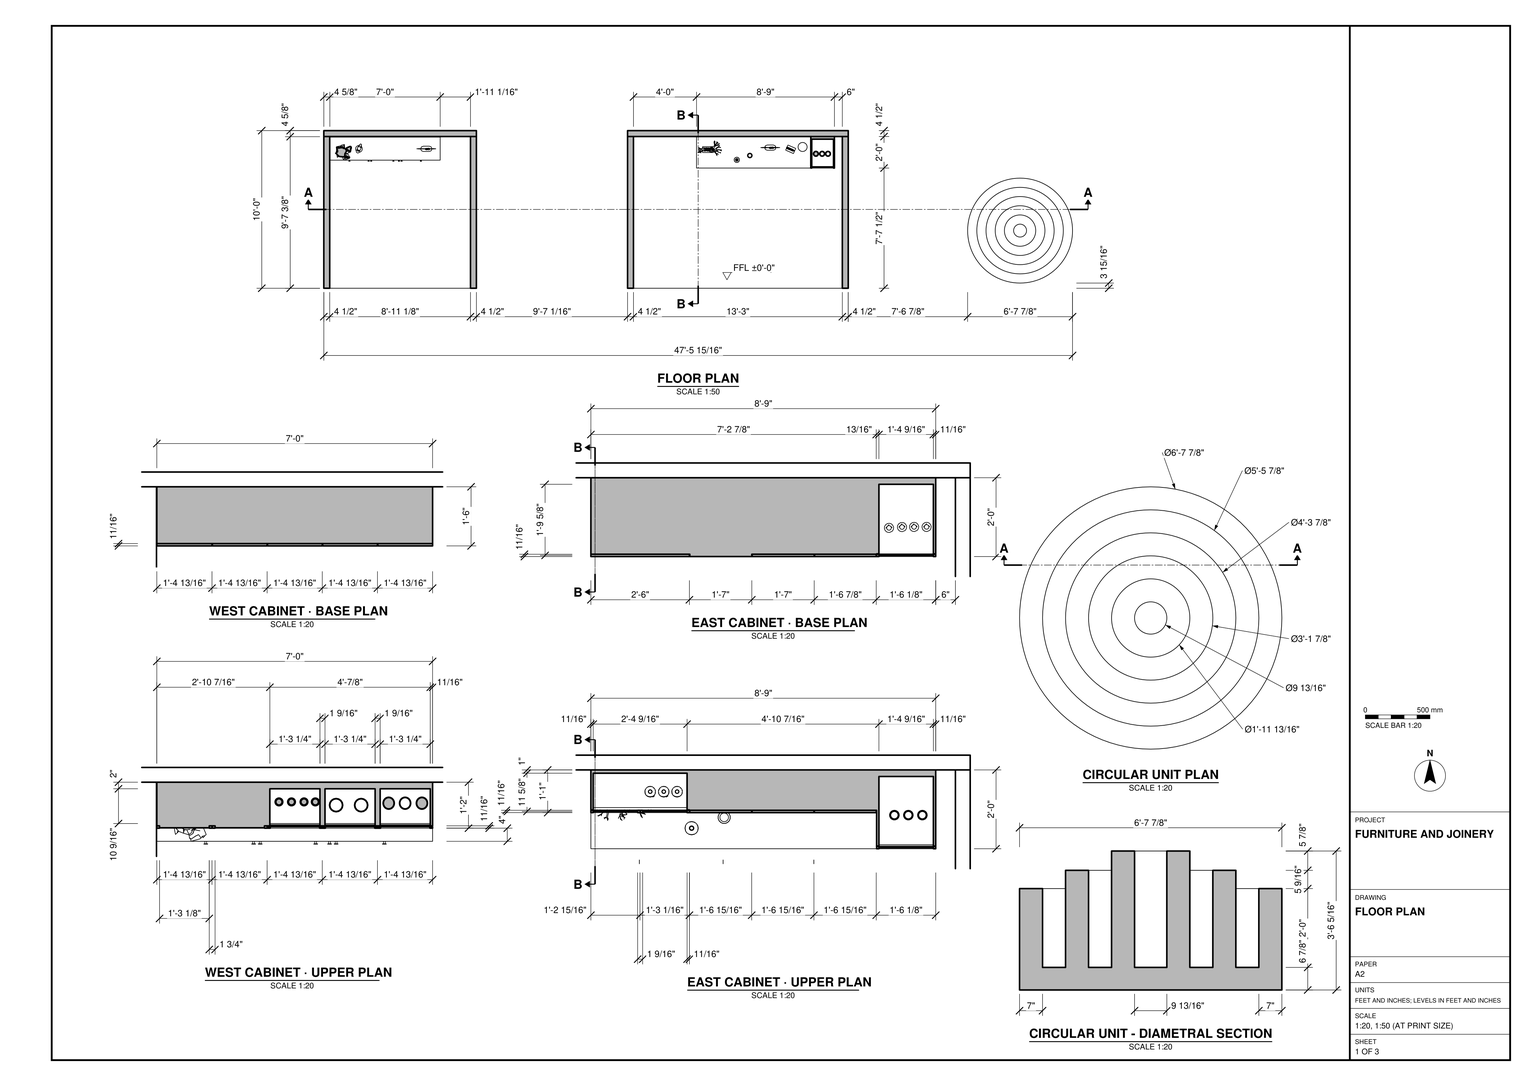
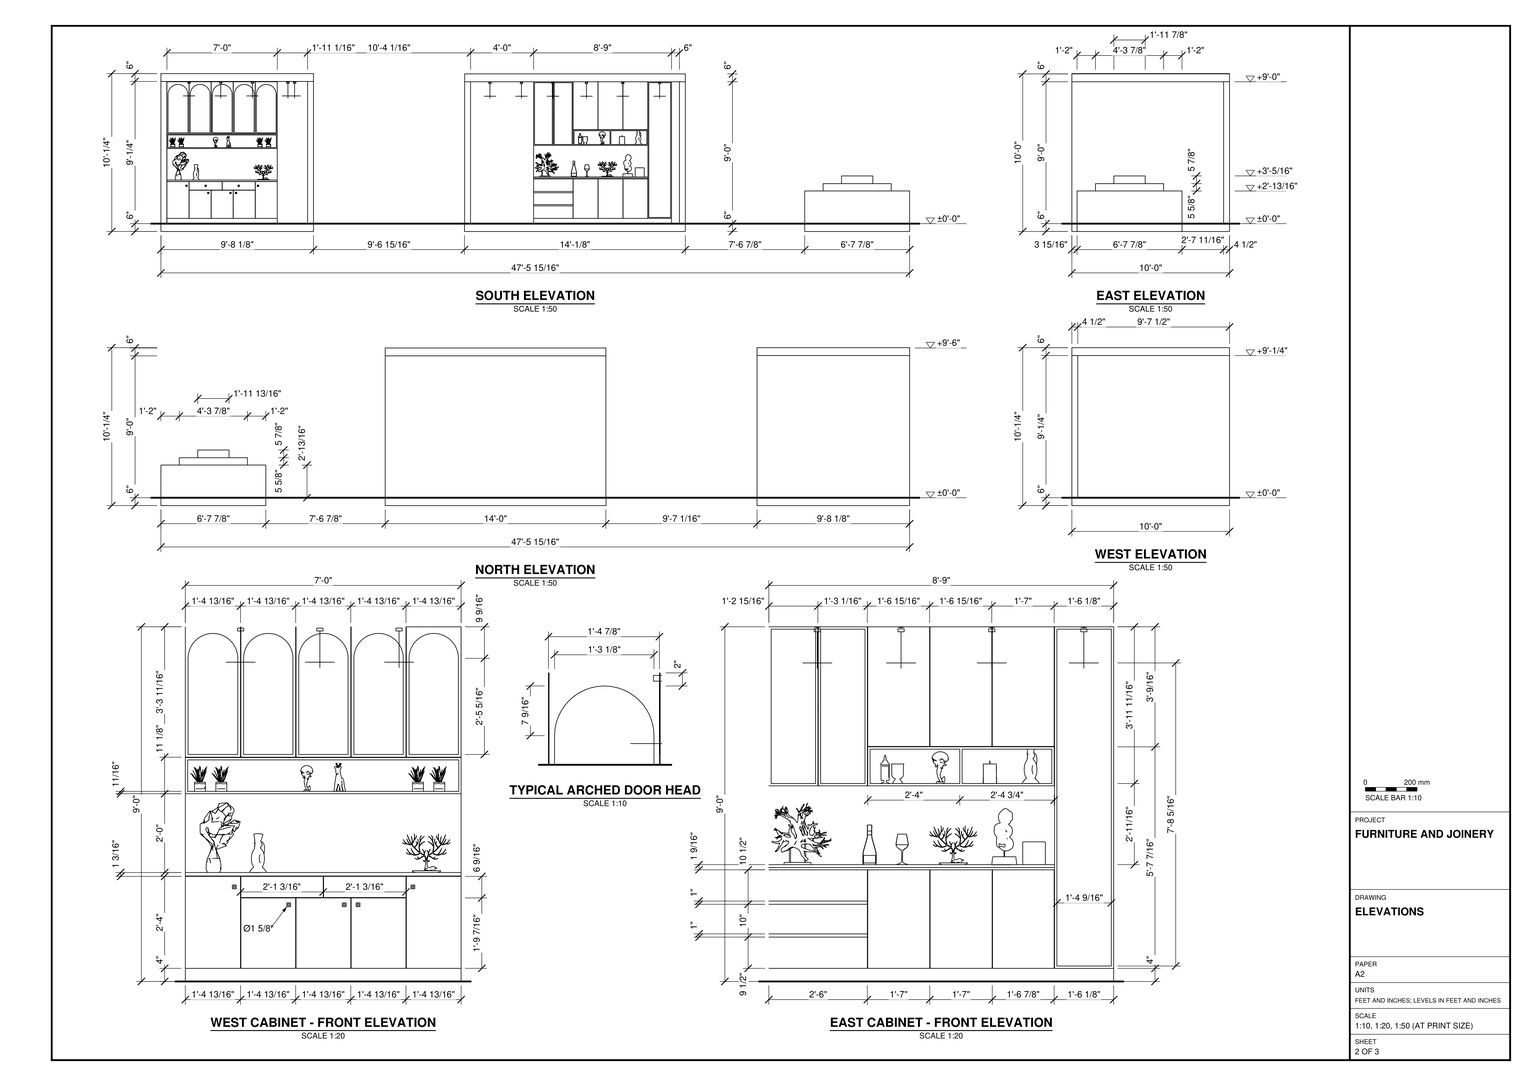
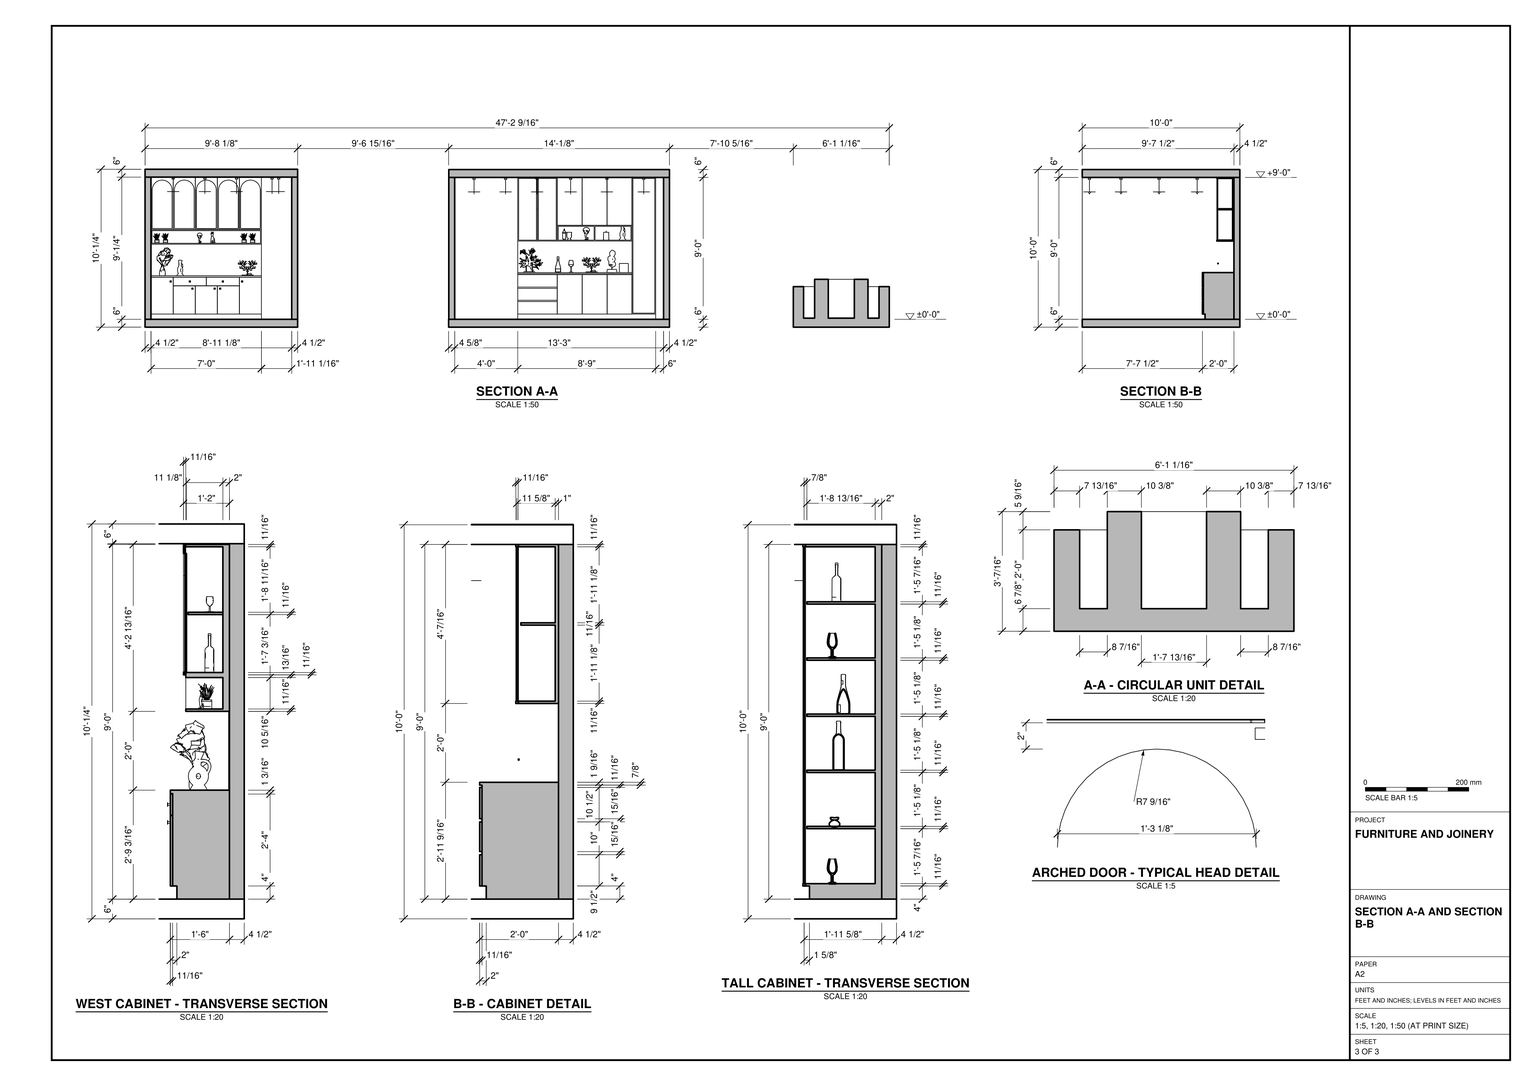
Work in feet and inches in SketchUp. Use task_files/diagram_01.pdf to model the west and east cabinet displays and the freestanding circular unit. Set the finished floor level to ±0'-0". The complete arrangement is 47'-5 15/16" long, 10'-0" deep and 10'-1/4" high.

Build each cabinet bay with a back wall, side walls, floor slab and overhead slab, leaving the south face open. Follow the wall and slab thicknesses in plan and section. Fit the 7'-0" west cabinet against the back wall at the left end of its bay. Model the recessed plinth, base doors and drawers, countertop, open display shelf and five arched upper door details. In the wider bay, leave 4'-0" of clear wall to the left of the 8'-9" east cabinet. Include the drawer bank, base doors, rectangular upper cupboards, open display compartments and full-height shelved cabinet at the right end.

Place the circular unit beyond the east bay. Use the diametral section to form its concentric walls on a common base, with open channels between the walls and the highest rim nearest the centre. Decor and loose items, including plants, bottles, glasses and ornaments, may be any suitable library components placed on the indicated counters and shelves.

Keep shell elements and each joinery piece in separate groups or components, and use components for repeated parts. Save one SketchUp model as output_files/two_cabinet_displays_and_freestanding_circular_unit.skp.

# SketchUp Ruby script. Lengths in inches.
U = 1.inch
M = Sketchup.active_model
def pt(a) = Geom::Point3d.new(a.map { |v| v * U })
def face(e, loops, mat)
  f = e.add_face(loops[0].map { |a| pt(a) })
  loops[1..].each { |l| e.add_face(l.map { |a| pt(a) }).erase! }
  f.material = f.back_material = mat if mat
  f
end
# faces: each face lists its corners as indices into pts; further lists are holes
def faces(e, pts, list, mat = nil) = list.each { |f| face(e, (f[0].is_a?(Array) ? f : [f]).map { |l| l.map { |i| pts[i] } }, mat) }
# xy, xz, yz: faces in a plane at the given z, y or x. An outline is a flat list of corners, or four numbers for a rectangle; further outlines are holes
def ring(l) = l.size == 4 ? [[l[0], l[1]], [l[2], l[1]], [l[2], l[3]], [l[0], l[3]]] : l.each_slice(2).to_a
def flat(e, list, mat, &to3) = list.each { |f| face(e, (f[0].is_a?(Array) ? f : [f]).map { |l| ring(l).map { |u, v| to3.(u, v) } }, mat) }
def xy(e, z, list, mat = nil) = flat(e, list, mat) { |x, y| [x, y, z] }
def xz(e, y, list, mat = nil) = flat(e, list, mat) { |x, z| [x, y, z] }
def yz(e, x, list, mat = nil) = flat(e, list, mat) { |y, z| [x, y, z] }
def lines(e, pts, list) = list.each { |a, b| e.add_line(pt(pts[a]), pt(pts[b])) }
# prism: a flat outline (further loops are holes) pulled along v
def prism(e, loops, v, mat = nil)
  f = face(e, loops, mat); d = Geom::Vector3d.new(v.map { |x| x * U })
  f.pushpull(f.normal.samedirection?(d) ? d.length : -d.length)
end
def box(e, o, s, mat = nil) = prism(e, [[o, [o[0] + s[0], o[1], o[2]], [o[0] + s[0], o[1] + s[1], o[2]], [o[0], o[1] + s[1], o[2]]]], [0, 0, s[2]], mat)
def at(x, y, z, deg = 0) = Geom::Transformation.translation(pt([x, y, z])) * Geom::Transformation.rotation(ORIGIN, Z_AXIS, deg.degrees)
def axes(o, x, y, z) = Geom::Transformation.new([*x, 0, *y, 0, *z, 0, *pt(o).to_a, 1])
def part(name) = M.definitions.add(name)
# library, detail: a bought-in or finely detailed component or shape, given as its bounding box
def library(name, o, s) = part(name).tap { |d| box(d.entities, o, s) }
def detail(e, o, s) = box(e.add_group.entities, o, s)
def put(e, d, t, mat = nil) = e.add_instance(d, t).tap { |i| i.material = mat if mat }
def group(e, t, mat = nil) = e.add_group.tap { |g| g.transformation = t; g.material = mat if mat }.entities
root = M.entities
M.materials.add("Sublime-734-Blanc-White-4K").color = [233, 236, 235]
M.materials.add("Sublime-735-Vert-Relax-Relax-Green-4K").color = [135, 152, 141]
M.materials.add("Uniboard-L17-Ambrette-4K").color = [104, 52, 49]
M.materials.add("Uniboard-L19-Putty-4K").color = [187, 181, 160]
M.materials.add("[Color M09]").color = [0, 0, 0]
M.materials.add("[Translucent Glass Gray]").color = [128, 128, 128]
M.materials["[Translucent Glass Gray]"].alpha = 0.5
c1 = library("Decoration 111 063",[-2.51,-1.28,-0.03],[5.02,2.53,10.66])
c2 = library("Interior Props 221 030",[-2.57,-3.63,-0.04],[5.13,7.27,11.89])
c3 = library("Decorative Jar 83-09",[-5.58,-3.02,0],[11.21,6.04,13.74])
c4 = library("Candle 111 040",[-2.11,-2.13,-0.02],[4.23,4.26,6.92])
c5 = library("Stand 298 006",[-6.74,-6.74,-0.04],[13.48,13.48,13.7])
c6 = library("Interior Props 221 024",[-3.28,-2.14,-0.05],[6.56,4.27,17.12])
c7 = library("Tree Decoration 83-10",[-18.61,-13.07,0],[43.1,29.04,44.77])
c8 = library("Decorative Deer 97-30",[-7.23,-2.03,0],[14.46,4,11.8125])
c9 = library("Wine Bottle 03 87-10",[-1.625,-1.66,0],[3.25,3.3,10.61])
c10 = library("Glass 002",[-1.85,-1.85,0.02],[3.7,3.7,9.27])
c11 = library("Bottle 05 87-12",[-2.04,-2.04,0],[4.08,4.08,12.09])
c12 = library("2-PRODUITS CUISINE CLC2",[-1.33,-1.33,0],[2.66,2.66,10.8])
c13 = library("16-PRODUITS CUISINE CLC2",[-2.49,-2.49,0],[4.98,4.98,4.3])
c14 = library("Vases 04 65-25",[-1.8125,-1.8125,0],[3.625,3.625,14.95])
c15 = part("Group39\#1")
p = [[0,0,0],[0,0,-2.67],[-1.27,0,-2.67],[8.29,-0.35,0],[-8.29,-0.35,0],[8.29,0.35,0],
  [8.29,0,0],[-8.29,0.35,0],[1.27,0,-2.67],[-8.29,0,0],[0,0,-4.32]]
lines(c15.entities,p,[[0,1],[1,2],[3,4],[5,6],[7,5],[1,8],[9,0],[0,6],[8,10],[4,9],[6,3],[2,10],
  [9,7]])
c16 = part("Rectangle Light")
put(c16.entities,c15,at(0,0,0))
c17 = part("Group41\#1")
p = [[0,0,0],[0,0,-13.54],[-6.68,0,-13.54],[43.5,-0.34,0],[-43.5,-0.34,0],[43.5,0.34,0],
  [43.5,0,0],[-43.5,0.34,0],[6.68,0,-13.54],[-43.5,0,0],[0,0,-21.92]]
lines(c17.entities,p,[[0,1],[1,2],[3,4],[5,6],[7,5],[1,8],[9,0],[0,6],[8,10],[4,9],[6,3],[2,10],
  [9,7]])
c18 = part("Rectangle Light\#1")
put(c18.entities,c17,at(0,0,0))
c19 = part("Group43\#1")
p = [[0,0,0],[0,0,-4.52],[-2.2,0,-4.52],[14.29,-0.35,0],[-14.29,-0.35,0],[14.29,0.35,0],
  [14.29,0,0],[-14.29,0.35,0],[2.2,0,-4.52],[-14.29,0,0],[0,0,-7.32]]
lines(c19.entities,p,[[0,1],[1,2],[3,4],[5,6],[7,5],[1,8],[9,0],[0,6],[8,10],[4,9],[6,3],[2,10],
  [9,7]])
c20 = part("Rectangle Light\#2")
put(c20.entities,c19,at(0,0,0))
c21 = part("Group45\#1")
p = [[0,0,0],[0,0,-4.33],[-2.1,0,-4.33],[13.66,-0.35,0],[-13.66,-0.35,0],[13.66,0.35,0],
  [13.66,0,0],[-13.66,0.35,0],[2.1,0,-4.33],[-13.66,0,0],[0,0,-7.01]]
lines(c21.entities,p,[[0,1],[1,2],[3,4],[5,6],[7,5],[1,8],[9,0],[0,6],[8,10],[4,9],[6,3],[2,10],
  [9,7]])
c22 = part("Rectangle Light\#3")
put(c22.entities,c21,at(0,0,0))
c23 = library("Wine 193 001",[-1.36,-1.37,-0.03],[2.74,2.77,11.85])
c24 = library("Wine Bottle 01 87-10",[-1.37,-1.39,0],[2.74,2.78,10.53])
c25 = library("Glass 298 004 004",[-1.29,-1.29,-0.01],[2.58,2.58,4.79])
c26 = part("Group68\#1")
p = [[0,0,0],[0,0,-2.47],[-1.17,0,-2.47],[7.63,-0.35,0],[-7.63,-0.35,0],[7.63,0.35,0],
  [7.63,0,0],[-7.63,0.35,0],[1.17,0,-2.47],[-7.63,0,0],[0,0,-3.99]]
lines(c26.entities,p,[[0,1],[1,2],[3,4],[5,6],[7,5],[1,8],[9,0],[0,6],[8,10],[4,9],[6,3],[2,10],
  [9,7]])
c27 = part("Rectangle Light\#4")
put(c27.entities,c26,at(0,0,0))
c28 = library("Interior Plant 273 003 001",[-15.3,-29.38,0],[45.32,44.44,78.66])
c29 = library("Decorative Deer 209 004",[-1.58,-4.16,0],[3.36,7.25,10.63])
c30 = library("Potted Succulent 003",[-4.09,-3.62,0],[7.1,6.83,10.79])
c31 = part("Group73\#1")
p = [[0,0,0],[0,0,-12.86],[-6.34,0,-12.86],[41.28,-0.35,0],[-41.28,-0.35,0],[41.28,0.35,0],
  [41.28,0,0],[-41.28,0.35,0],[6.34,0,-12.86],[-41.28,0,0],[0,0,-20.82]]
lines(c31.entities,p,[[0,1],[1,2],[3,4],[5,6],[7,5],[1,8],[9,0],[0,6],[8,10],[4,9],[6,3],[2,10],
  [9,7]])
c32 = part("Rectangle Light\#5")
put(c32.entities,c31,at(0,0,0))
c33 = library("031",[-37.9375,-66.55,25.1875],[1.17,0.87,1.16])
c34 = library("Wine Glass 293 011",[-1.4,-1.42,-0.1],[2.82,2.8,7.63])
c35 = library("Group\#6",[0,0,0],[8.9,8.9,12.63])
c36 = part("Group\#8")
box(c36.entities,[3.84,0,0],[116.16,120,6])
c37 = library("Group\#11",[0,4,0],[83.97,14,50.82])
c38 = library("Group\#18",[0,0,0],[8.9,8.9,12.63])
xz(root,91.85,[[371.43,10.71,388.01,113.29]],"[Translucent Glass Gray]")
detail(root,[490.09,3.96,0],[79.88,79.87,42.3125])
put(root,c1,axes([335.9,107.74,66.28],[1,0,0],[0,1,0],[0,0,0.91]))
put(root,c2,at(363.56,107.74,66.28,-21.7))
put(root,c3,axes([321.28,107.85,66.28],[0.63,0,0],[0,0.63,0],[0,0,0.63]))
put(root,c4,at(351.03,106.9,66.28))
put(root,c5,axes([364.47,107.5625,41.55],[0.51,0,0],[0,0.51,0],[0,0,0.51]))
put(root,c6,at(355.37,105.8125,41.57,-23.6))
put(root,c7,axes([292.47,105.56,41.57],[0.42,0,0],[0,0.42,0],[0,0,0.42]))
put(root,c8,at(339.87,107.08,41.57))
put(root,c9,at(309.96,108.875,90.14))
put(root,c9,at(305.9,108.875,90.14))
put(root,c9,at(301.77,108.875,90.14))
put(root,c10,at(324.31,101.05,41.57))
put(root,c11,at(314.39,97.76,41.57))
put(root,c11,at(384.35,103.82,62.35))
put(root,c11,at(379.41,103.82,62.35))
put(root,c11,at(374.35,103.82,62.35))
put(root,c12,at(287.78,109.78,90.14))
put(root,c12,at(291.4,109.78,90.14))
put(root,c12,at(295.03,109.78,90.14))
put(root,c13,at(376.64,101.11,27.63))
put(root,c13,at(383.33,101.11,27.63))
put(root,c14,at(379.35,102.37,45.26))
put(root,c14,at(374.6,102.37,45.26))
put(root,c14,at(383.79,102.37,45.26))
put(root,c16,axes([379.72,112.4375,113.28],[1,0,0],[0,-1,0],[0,0,1]))
put(root,c16,axes([379.72,112.4375,95.84],[1,0,0],[0,-1,0],[0,0,1]))
put(root,c16,axes([379.72,112.4375,78.74],[1,0,0],[0,-1,0],[0,0,1]))
put(root,c16,axes([379.72,112.4375,61.65],[1,0,0],[0,-1,0],[0,0,1]))
put(root,c16,axes([379.72,112.4375,44.55],[1,0,0],[0,-1,0],[0,0,1]))
put(root,c16,axes([379.72,112.4375,27.45],[1,0,0],[0,-1,0],[0,0,1]))
put(root,c18,at(327.22,114.45,65.56,180))
put(root,c20,at(298.72,112.4375,113.28,180))
put(root,c20,at(298.72,112.4375,89.42,180))
put(root,c22,axes([328.2,113.4375,76.74],[1,0,0],[0,-1,0],[0,0,1]))
put(root,c22,axes([356.23,113.4375,76.74],[1,0,0],[0,-1,0],[0,0,1]))
put(root,c23,at(41.98,109.39,75.01))
put(root,c23,at(46.36,109.39,75.01))
put(root,c23,at(50.79,109.39,75.01))
put(root,c24,at(58.8,108.51,75.01))
put(root,c24,at(63.68,108.51,75.01))
put(root,c24,at(68.43,108.51,75.01))
put(root,c9,at(75.77,109.55,75.01))
put(root,c9,at(80.2,109.55,75.01))
put(root,c9,at(85.08,109.55,75.01))
put(root,c25,at(41.79,109.5,93.36))
put(root,c25,at(45.61,109.5,93.36))
put(root,c25,at(49.42,109.5,93.36))
put(root,c25,at(52.86,109.5,93.36))
put(root,c14,axes([75.21,109.11,93.36],[0.94,0,0],[0,1,0],[0,0,0.89]))
put(root,c14,axes([80.2,109.11,93.36],[0.94,0,0],[0,1,0],[0,0,0.89]))
put(root,c14,axes([85.32,109.11,93.36],[0.94,0,0],[0,1,0],[0,0,0.89]))
put(root,c11,at(59.19,108.51,93.36))
put(root,c11,at(66.82,108.51,93.36))
put(root,c27,at(46.65,106.69,113.28,180))
put(root,c27,at(63.44,105.88,113.28,180))
put(root,c27,at(80.24,105.38,113.28,180))
put(root,c27,at(80.24,105.94,92.64,180))
put(root,c27,at(46.65,107.69,92.64,180))
put(root,c27,at(63.44,105.94,92.64,180))
put(root,c28,axes([13.22,105.43,39.18],[0.27,0,0],[0,0.27,0],[0,0,0.27]))
put(root,c1,axes([41.57,107.05,63.88],[0.74,0,0],[0,0.74,0],[0,0,0.74]))
put(root,c2,at(26.85,106.41,39.18,-23.2))
put(root,c29,axes([51.47,108.15,63.89],[0.7824,-0.20964,0],[0.20964,0.7824,0],[0,0,0.81]))
put(root,c8,at(78.01,106.17,39.18))
put(root,c30,axes([9.08,108.55,63.89],[0.71,0,0],[0,0.71,0],[0,0,0.71]))
put(root,c30,axes([15.58,108.55,63.89],[0.71,0,0],[0,0.71,0],[0,0,0.71]))
put(root,c30,axes([75.46,108.55,63.89],[0.71,0,0],[0,0.71,0],[0,0,0.71]))
put(root,c30,axes([81.96,108.55,63.89],[0.71,0,0],[0,0.71,0],[0,0,0.71]))
put(root,c32,axes([46.59,112.4375,73.46],[1,0,0],[0,-1,0],[0,0,1]))
put(root,c32,axes([47.3,114.4375,63.17],[1,0,0],[0,-1,0],[0,0,1]))
put(root,c33,at(71.43,163.18,9.03))
put(root,c33,at(96.55,163.18,9.03))
put(root,c33,at(94.55,163.18,3.59))
put(root,c33,at(73.43,163.18,3.59))
put(root,c33,at(90.33,163.18,3.59))
put(root,c33,at(111.24,163.18,9.03))
put(root,c33,at(56.86,163.18,9.03))
g1 = group(root,at(279.22,0,0))
box(g1,[-48.12,0,0],[168.12,120,6])
g2 = group(root,at(279.22,115.5,6))
xy(g2,0,[[-47.99,0,120,4.5]])
xy(g2,108,[[-47.99,0,120,4.5]])
xz(g2,0,[[-47.99,0,4.5,108],[4.5,0,115.5,0,115.5,108,4.5,108,4.5,59.57,91.5,59.57,91.5,35.57,4.5,35.57],[115.5,0,120,108],[4.5,35.57,91.5,59.57]])
xz(g2,4.5,[[-47.99,0,120,108]])
yz(g2,-47.99,[[0,0,4.5,108]])
yz(g2,120,[[0,0,4.5,108]])
g3 = group(root,at(283.72,91.5,6),"Uniboard-L19-Putty-4K")
xy(g3,0,[[0,2,87,24],[87,2,105,24]])
xy(g3,4,[[0,0,30,0.71],[30.12,0,49,0.71],[49.12,0,68,0.71],[68.12,0,86.88,0.71],[87,0,105,0.71],
  [0,0.71,30,2],[30,0.71,49,2],[49,0.71,68,2],[68,0.71,87,2],[87,0.83,105,2]])
xy(g3,4.71,[[87.71,0.83,104.29,22]],"Uniboard-L17-Ambrette-4K")
xy(g3,4.71,[[87.71,0,104.29,0.71]],"[Color M09]")
xy(g3,13.51,[[0,0,30,0.71]],"[Color M09]")
xy(g3,14.49,[[0,0,30,0.71]],"[Color M09]")
xy(g3,21.45,[[87.71,1.22,104.29,22]],"Uniboard-L17-Ambrette-4K")
xy(g3,22.16,[[87.71,1.22,104.29,22]],"Uniboard-L17-Ambrette-4K")
xy(g3,23.51,[[0,0,30,0.71]],"[Color M09]")
xy(g3,24.49,[[0,0,30,0.71]],"[Color M09]")
xy(g3,34,[[0,0,30,0.71],[30.12,0,49,0.71],[49.12,0,68,0.71],[68.12,0,86.88,0.71]])
xy(g3,34.71,[[0,0,87,0.71]])
xy(g3,35.57,[[0,0,87,24]])
xy(g3,38.55,[[87.71,1.22,104.29,22]],"Uniboard-L17-Ambrette-4K")
xy(g3,39.26,[[87.71,1.22,104.29,22]],"Uniboard-L17-Ambrette-4K")
xy(g3,55.65,[[87.71,1.22,104.29,22]],"Uniboard-L17-Ambrette-4K")
xy(g3,56.35,[[87.71,1.22,104.29,22]],"Uniboard-L17-Ambrette-4K")
xy(g3,59.57,[[0,11,14.94,11.71],[15.06,11,30,11.71],[30.12,11.52,30.12,11.71,30,11.71,30,11.83,0,11.83,0,24,87,24,87,11.71,86.88,11.71,86.88,11.52]])
xy(g3,60.28,[[30.83,11.52,58.15,23],[58.85,11.52,86.17,23],[0.71,11.83,29.29,23]],"Uniboard-L17-Ambrette-4K")
xy(g3,60.28,[[0.71,11,14.23,11.35],[15.77,11,29.29,11.35],[0.71,11.35,14.23,11.71],[15.77,11.35,29.29,11.71]],"[Color M09]")
xy(g3,70.75,[[30.83,11.52,58.15,23],[58.85,11.52,86.17,23]],"Uniboard-L17-Ambrette-4K")
xy(g3,71.46,[[67.92,11.52,68.04,11.71]])
xy(g3,71.46,[[30.12,11.52,48.96,11.71],[48.96,11.52,49.08,11.71],[49.08,11.52,67.92,11.71],[68.04,11.52,86.88,11.71]],"Uniboard-L17-Ambrette-4K")
xy(g3,71.57,[[30.12,11,48.96,11.71],[49.08,11,67.92,11.71],[68.04,11,86.88,11.71]])
xy(g3,72.74,[[87.71,1.22,104.29,22]],"Uniboard-L17-Ambrette-4K")
xy(g3,73.45,[[87.71,1.22,104.29,22]],"Uniboard-L17-Ambrette-4K")
xy(g3,83.43,[[0.71,12.54,29.29,23]],"Uniboard-L17-Ambrette-4K")
xy(g3,84.14,[[0.71,12.54,29.29,23]],"Uniboard-L17-Ambrette-4K")
xy(g3,89.84,[[87.71,1.22,104.29,22]],"Uniboard-L17-Ambrette-4K")
xy(g3,90.55,[[87.71,1.22,104.29,22]],"Uniboard-L17-Ambrette-4K")
xy(g3,107.29,[[87.71,0.83,104.29,22],[0.71,11.83,29.29,23]],"Uniboard-L17-Ambrette-4K")
xy(g3,107.29,[[87.71,0,104.29,0.71],[0.71,11,14.23,11.35],[15.77,11,29.29,11.35],[0.71,11.35,14.23,11.71],[15.77,11.35,29.29,11.71]],"[Color M09]")
xy(g3,108,[[87,0.83,105,0.83,105,24,0,24,0,11.83,30,11.83,30,11.71,87,11.71],[30.12,11,48.96,11.71],[49.08,11,67.92,11.71],[68.04,11,86.88,11.71]])
xy(g3,108,[[87,0,105,0.71],[0,11,14.94,11.71],[15.06,11,30,11.71]],"[Color M09]")
xz(g3,0,[[0,4,30,13.51],[30.12,4,49,34],[49.12,4,68,34],[68.12,4,86.88,34],[0,14.49,30,23.51],
  [0,24.49,30,34],[0,34.71,87,35.57]])
xz(g3,0,[[[87,4,105,108],[87.71,4.71,104.29,107.29]]],"[Color M09]")
xz(g3,0.71,[[0,4,30,13.51],[30,4,30.12,34],[49,4,49.12,34],[49.12,4,68,34],[68,4,68.12,34],
  [68.12,4,86.88,34],[86.88,4,87,34],[87,4,104.29,4.71],[104.29,4,105,108],[87,4.71,87.71,107.29],
  [0,14.49,30,23.51],[0,24.49,30,34],[87,107.29,104.29,108]])
xz(g3,0.71,[[0,13.51,30,14.49],[0,23.51,30,24.49],[0,34,87,34.71]],"[Color M09]")
xz(g3,0.83,[[87,4,104.29,4.71],[104.29,4,105,108],[87,4.71,87.71,107.29],[87,107.29,104.29,108]],"Uniboard-L17-Ambrette-4K")
xz(g3,1.22,[[87.71,21.45,104.29,22.16],[87.71,38.55,104.29,39.26],[87.71,55.65,104.29,56.35],[87.71,72.74,104.29,73.45],[87.71,89.84,104.29,90.55]],"Uniboard-L17-Ambrette-4K")
xz(g3,2,[[0,0,105,4]])
xz(g3,11,[[30.12,71.57,48.96,108],[68.04,71.57,86.88,108]])
xz(g3,11,[[49.08,71.57,67.92,108]],"Uniboard-L19-Putty-4K")
xz(g3,11,[[[0,59.57,14.94,108],[0.71,60.28,14.23,107.29]],[[15.06,59.57,30,108],[15.77,60.28,29.29,107.29]]],"[Color M09]")
xz(g3,11.35,[[0.71,60.28,14.23,107.29],[15.77,60.28,29.29,107.29]],"[Translucent Glass Gray]")
xz(g3,11.52,[[[30.12,59.57,86.88,71.46],[30.83,60.28,58.15,70.75],[58.85,60.28,86.17,70.75]]],"Uniboard-L17-Ambrette-4K")
xz(g3,11.71,[[0,59.57,0.71,108],[0.71,59.57,14.94,60.28],[15.06,59.57,30,60.28],[30,59.57,30.12,108],[86.88,59.57,87,108],
  [14.23,60.28,14.23,107.29,0.71,107.29,0.71,108,14.94,108,14.94,60.28],[15.06,60.28,15.06,108,29.29,108,29.29,107.29,15.77,107.29,15.77,60.28],[29.29,60.28,30,108],[30.12,71.46,86.88,71.57],[30.12,71.57,48.96,108],
  [48.96,71.57,49.08,108],[49.08,71.57,67.92,108],[67.92,71.57,68.04,108],[68.04,71.57,86.88,108]])
xz(g3,11.83,[[0,59.57,30,59.57,30,60.28,0.71,60.28,0.71,107.29,29.29,107.29,29.29,60.28,30,60.28,30,108,0,108]],"Uniboard-L17-Ambrette-4K")
xz(g3,12.54,[[0.71,83.43,29.29,84.14]],"Uniboard-L17-Ambrette-4K")
xz(g3,22,[[87.71,4.71,104.29,21.45],[87.71,22.16,104.29,38.55],[87.71,39.26,104.29,55.65],[87.71,56.35,104.29,72.74],[87.71,73.45,104.29,89.84],
  [87.71,90.55,104.29,107.29]],"Uniboard-L17-Ambrette-4K")
xz(g3,23,[[0.71,60.28,29.29,83.43],[30.83,60.28,58.15,70.75],[58.85,60.28,86.17,70.75],[0.71,84.14,29.29,107.29]],"Uniboard-L17-Ambrette-4K")
xz(g3,24,[[0,0,87,34],[87,0,87,59.57,0,59.57,0,108,105,108,105,0],[0,34,87,35.57]])
yz(g3,0,[[2,0,2,4,0.71,4,0.71,34.71,24,34.71,24,0],[0,4,0.71,13.51],[0,14.49,0.71,23.51],[0,24.49,0.71,34],[0,34.71,24,35.57],
  [11.83,59.57,24,108]])
yz(g3,0,[[11,59.57,11.71,108]],"[Color M09]")
yz(g3,0.71,[[11.83,60.28,23,60.28,23,83.43,12.54,83.43,12.54,84.14,23,84.14,23,107.29,11.83,107.29]],"Uniboard-L17-Ambrette-4K")
yz(g3,0.71,[[11,60.28,11.35,107.29],[11.35,60.28,11.71,107.29]],"[Color M09]")
yz(g3,14.23,[[11,60.28,11.35,107.29],[11.35,60.28,11.71,107.29]],"[Color M09]")
yz(g3,14.94,[[11,59.57,11.71,108]],"[Color M09]")
yz(g3,15.06,[[11,59.57,11.71,108]],"[Color M09]")
yz(g3,15.77,[[11,60.28,11.35,107.29],[11.35,60.28,11.71,107.29]],"[Color M09]")
yz(g3,29.29,[[11.83,60.28,11.83,107.29,23,107.29,23,84.14,12.54,84.14,12.54,83.43,23,83.43,23,60.28]],"Uniboard-L17-Ambrette-4K")
yz(g3,29.29,[[11,60.28,11.35,107.29],[11.35,60.28,11.71,107.29]],"[Color M09]")
yz(g3,30,[[0,4,0.71,13.51],[0,14.49,0.71,23.51],[0,24.49,0.71,34],[11.71,59.57,11.83,108]])
yz(g3,30,[[11,59.57,11.71,108]],"[Color M09]")
yz(g3,30.12,[[0,4,0.71,34],[11.52,59.57,11.71,71.46],[11,71.57,11.71,108]])
yz(g3,30.83,[[11.52,60.28,23,70.75]],"Uniboard-L17-Ambrette-4K")
yz(g3,48.96,[[11,71.57,11.71,108]])
yz(g3,49,[[0,4,0.71,34]])
yz(g3,49.08,[[11,71.57,11.71,108]])
yz(g3,49.12,[[0,4,0.71,34]])
yz(g3,58.15,[[11.52,60.28,23,70.75]],"Uniboard-L17-Ambrette-4K")
yz(g3,58.85,[[11.52,60.28,23,70.75]],"Uniboard-L17-Ambrette-4K")
yz(g3,67.92,[[11,71.57,11.71,108]])
yz(g3,68,[[0,4,0.71,34]])
yz(g3,68.04,[[11,71.57,11.71,108]])
yz(g3,68.12,[[0,4,0.71,34]])
yz(g3,86.17,[[11.52,60.28,23,70.75]],"Uniboard-L17-Ambrette-4K")
yz(g3,86.88,[[0,4,0.71,34],[11,71.57,11.71,108]])
yz(g3,86.88,[[11.52,59.57,11.71,71.46]],"Uniboard-L17-Ambrette-4K")
yz(g3,87,[[0,4,0.71,34],[0.71,4,0.83,34],[0,34,0.71,34.71],[0.71,34,0.83,35.57],[0.83,34,24,35.57],
  [0,34.71,0.71,35.57],[0.71,35.57,0.83,108],[0.83,35.57,0.83,108,11.71,108,11.71,59.57,24,59.57,24,35.57]])
yz(g3,87,[[0,35.57,0.71,108]],"[Color M09]")
yz(g3,87.71,[[0.83,4.71,22,4.71,22,21.45,1.22,21.45,1.22,22.16,22,22.16,22,38.55,1.22,38.55,1.22,39.26,22,39.26,22,55.65,1.22,55.65,1.22,56.35,22,56.35,22,72.74,1.22,72.74,1.22,73.45,22,73.45,22,89.84,1.22,89.84,1.22,90.55,22,90.55,22,107.29,0.83,107.29]],"Uniboard-L17-Ambrette-4K")
yz(g3,87.71,[[0,4.71,0.71,107.29]],"[Color M09]")
yz(g3,104.29,[[0.83,4.71,0.83,107.29,22,107.29,22,90.55,1.22,90.55,1.22,89.84,22,89.84,22,73.45,1.22,73.45,1.22,72.74,22,72.74,22,56.35,1.22,56.35,1.22,55.65,22,55.65,22,39.26,1.22,39.26,1.22,38.55,22,38.55,22,22.16,1.22,22.16,1.22,21.45,22,21.45,22,4.71]],"Uniboard-L17-Ambrette-4K")
yz(g3,104.29,[[0,4.71,0.71,107.29]],"[Color M09]")
yz(g3,105,[[2,0,24,0,24,108,0.83,108,0.83,4,2,4]])
yz(g3,105,[[0,4,0.71,108]],"[Color M09]")
put(g3,c23,at(26.86,17.26,60.28))
put(g3,c34,at(3.14,17.62,60.28))
put(g3,c34,at(6.98,17.87,60.28))
put(g3,c34,at(10.34,17.91,60.28))
put(g3,c23,at(22.59,17.26,60.28))
put(g3,c23,at(18.34,17.26,60.28))
put(g3,c34,at(94.73,8.99,4.71))
put(g3,c34,at(98.41,9.02,4.71))
put(g3,c34,at(90.77,8.73,4.71))
put(g3,c34,at(102.22,9.02,4.71))
put(g3,c23,at(100.93,10.21,90.55))
put(g3,c23,at(92.41,10.21,90.55))
put(g3,c23,at(96.66,10.21,90.55))
put(g3,c34,at(98.41,9.02,73.45))
put(g3,c34,at(94.73,8.99,73.45))
put(g3,c34,at(90.77,8.73,73.45))
put(g3,c34,at(102.22,9.02,73.45))
g4 = group(root,at(231.22,0,6))
box(g4,[0,0,0],[4.5,115.5,108])
g5 = group(root,at(394.72,0,6))
box(g5,[0,0,0],[4.5,115.5,108])
g6 = group(root,at(279.22,0,114))
box(g6,[-47.99,0,0],[167.99,120,6])
put(root,c35,at(294.02,83.05,101.37))
put(root,c35,at(319.53,83.05,101.37))
put(root,c35,at(347.16,83.05,101.37))
put(root,c35,at(375.19,70.25,101.37))
put(root,c35,at(347.16,54.05,101.37))
put(root,c35,at(319.53,54.05,101.37))
put(root,c35,at(294.02,54.05,101.37))
put(root,c35,at(347.16,25.05,101.37))
put(root,c35,at(319.53,25.05,101.37))
put(root,c35,at(294.02,25.05,101.37))
put(root,c35,at(347.16,1.05,101.37))
put(root,c35,at(319.53,1.05,101.37))
put(root,c35,at(294.02,1.05,101.37))
put(root,c35,at(375.19,46.25,101.37))
put(root,c35,at(375.19,22.25,101.37))
put(root,c35,at(375.19,2.44,101.37))
put(root,c35,at(270.02,1.05,101.37))
put(root,c35,at(270.02,25.05,101.37))
put(root,c35,at(270.02,83.05,101.37))
put(root,c35,at(270.02,54.05,101.37))
put(root,c35,at(246.02,1.05,101.37))
put(root,c35,at(246.02,25.05,101.37))
put(root,c35,at(246.02,83.05,101.37))
put(root,c35,at(246.02,54.05,101.37))
put(root,c35,at(246.02,103.05,101.37))
put(root,c35,at(270.02,103.05,101.37))
put(root,c36,at(-3.84,0,0))
g7 = group(root,at(-3.84,115.5,6))
xy(g7,0,[[3.84,0,120,4.5]])
xy(g7,33.18,[[8.44,-0.12,92.42,0]])
xy(g7,57.18,[[8.44,-0.12,92.42,0]])
xy(g7,108.24,[[3.84,0,120,4.5]])
xz(g7,-0.12,[[8.44,33.18,92.42,57.18]])
xz(g7,0,[[[3.84,0,120,108.24],[8.44,33.18,92.42,57.18]],[8.44,33.18,92.42,57.18]])
xz(g7,4.5,[[3.84,0,120,108.24]])
yz(g7,3.84,[[0,0,4.5,108.24]])
yz(g7,8.44,[[-0.12,33.18,0,57.18]])
yz(g7,92.42,[[-0.12,33.18,0,57.18]])
yz(g7,120,[[0,0,4.5,108.24]])
g8 = group(root,at(4.6,97.5,6),"Sublime-734-Blanc-White-4K")
xy(g8,0,[[0,2,83.97,18]])
xy(g8,4,[[0,0,16.79,0.71],[16.91,0,33.59,0.71],[33.71,0,50.38,0.71],[50.5,0,67.18,0.71],[67.3,0,83.97,0.71],
  [0,0.71,83.97,2]])
xy(g8,25.44,[[16.91,0,33.59,0.71],[33.71,0,50.38,0.71],[50.5,0,67.18,0.71]])
xy(g8,25.56,[[16.91,0,41.99,0.71],[42.11,0,67.18,0.71]])
xy(g8,32,[[0,0,16.79,0.71],[16.91,0,33.59,0.71],[33.59,0,41.99,0.71],[42.11,0,50.38,0.71],[50.38,0,67.18,0.71],
  [67.3,0,83.97,0.71]])
xy(g8,32.12,[[0,0,83.97,0.71]],"Sublime-735-Vert-Relax-Relax-Green-4K")
xy(g8,33.18,[[0,0,83.97,18]],"Sublime-735-Vert-Relax-Relax-Green-4K")
xz(g8,0,[[0,4,16.79,32],[16.91,4,33.59,25.44],[33.71,4,50.38,25.44],[50.5,4,67.18,25.44],[67.3,4,83.97,32],
  [16.91,25.56,41.99,32],[42.11,25.56,67.18,32]])
xz(g8,0,[[0,32.12,83.97,33.18]],"Sublime-735-Vert-Relax-Relax-Green-4K")
xz(g8,0.71,[[0,4,16.79,32],[16.79,4,16.91,32],[16.91,4,33.59,25.44],[33.59,4,33.71,25.44],[33.71,4,50.38,25.44],
  [50.38,4,50.5,25.44],[50.5,4,67.18,25.44],[67.18,4,67.3,32],[67.3,4,83.97,32],[16.91,25.44,67.18,25.44,67.18,25.56,42.11,25.56,42.11,32,41.99,32,41.99,25.56,16.91,25.56],
  [16.91,25.56,41.99,32],[42.11,25.56,67.18,32],[0,32,83.97,32.12]])
xz(g8,2,[[0,0,83.97,4]],"Sublime-735-Vert-Relax-Relax-Green-4K")
xz(g8,18,[[0,0,83.97,32],[0,32,83.97,33.18]])
yz(g8,0,[[2,0,2,4,0.71,4,0.71,32.12,18,32.12,18,0],[0,4,0.71,32],[0,32.12,18,33.18]])
yz(g8,16.79,[[0,4,0.71,25.44],[0,25.44,0.71,32]])
yz(g8,16.91,[[0,4,0.71,25.44],[0,25.56,0.71,32]])
yz(g8,33.59,[[0,4,0.71,25.44]])
yz(g8,33.71,[[0,4,0.71,25.44]])
yz(g8,41.99,[[0,25.56,0.71,32]])
yz(g8,42.11,[[0,25.56,0.71,32]])
yz(g8,50.38,[[0,4,0.71,25.44]])
yz(g8,50.5,[[0,4,0.71,25.44]])
yz(g8,67.18,[[0,4,0.71,25.44],[0,25.56,0.71,32]])
yz(g8,67.3,[[0,4,0.71,32]])
yz(g8,83.97,[[2,0,18,0,18,32.12,0.71,32.12,0.71,4,2,4],[0,4,0.71,32]])
yz(g8,83.97,[[0,32.12,18,33.18]],"Sublime-735-Vert-Relax-Relax-Green-4K")
put(root,c37,at(4.6,97.5,63.18),"Sublime-735-Vert-Relax-Relax-Green-4K")
g9 = group(root,at(39.02,102.92,92.65),"Sublime-735-Vert-Relax-Relax-Green-4K")
box(g9,[0,0,0],[15.26,10.58,0.71])
box(g9,[33.59,0,0],[15.26,10.58,0.71])
xy(g9,0,[[16.79,0,32.05,10.58]],"Sublime-735-Vert-Relax-Relax-Green-4K")
xy(g9,0.71,[[16.79,0,32.05,10.58]],"Sublime-735-Vert-Relax-Relax-Green-4K")
xz(g9,0,[[16.79,0,32.05,0.71]],"Sublime-735-Vert-Relax-Relax-Green-4K")
xz(g9,10.58,[[16.79,0,32.05,0.71]])
yz(g9,16.79,[[0,0,10.58,0.71]])
yz(g9,32.05,[[0,0,10.58,0.71]])
g10 = group(root,at(0,0,6))
box(g10,[0,0,0],[4.5,115.5,108.24])
g11 = group(root,at(38.31,101.5,74.3),"Sublime-735-Vert-Relax-Relax-Green-4K")
xy(g11,0,[[0,0,16.68,0.46]])
xy(g11,0.83,[[0.83,0,15.85,0.92]])
xy(g11,39.7,[[0,0,16.68,0.46]])
xz(g11,0,[[[0,0,16.68,39.7],[0.83,0.83,15.85,0.83,15.85,30.1875,15.79,31.17,15.59,32.13,15.28,33.0625,14.84,33.95,14.3,34.76,13.65,35.5,12.91,36.15,12.09,36.69,11.21,37.13,10.28,37.44,9.32,37.64,8.34,37.7,7.36,37.64,6.39,37.44,5.46,37.13,4.58,36.69,3.77,36.15,3.03,35.5,2.38,34.76,1.83,33.95,1.4,33.0625,1.08,32.13,0.89,31.17,0.83,30.1875]]])
xz(g11,0.46,[[0,0,16.68,39.7]],"[Translucent Glass Gray]")
xz(g11,0.92,[[0.83,0.83,0.83,30.1875,0.89,31.17,1.08,32.13,1.4,33.0625,1.83,33.95,2.38,34.76,3.03,35.5,3.77,36.15,4.58,36.69,5.46,37.13,6.39,37.44,7.36,37.64,8.34,37.7,9.32,37.64,10.28,37.44,11.21,37.13,12.09,36.69,12.91,36.15,13.65,35.5,14.3,34.76,14.84,33.95,15.28,33.0625,15.59,32.13,15.79,31.17,15.85,30.1875,15.85,0.83]],"[Translucent Glass Gray]")
yz(g11,0,[[0,0,0.46,39.7]])
yz(g11,0.83,[[0,0.83,0.92,30.1875]])
yz(g11,15.85,[[0,0.83,0.92,30.1875]])
yz(g11,16.68,[[0,0,0.46,39.7]])
p = [[0.83,0,30.1875],[0.89,0,31.17],[0.89,0.92,31.17],[0.83,0.92,30.1875],[15.79,0,31.17],[15.85,0,30.1875],
  [15.85,0.92,30.1875],[15.79,0.92,31.17],[1.08,0,32.13],[1.08,0.92,32.13],[15.59,0,32.13],[15.59,0.92,32.13],
  [1.4,0,33.0625],[1.4,0.92,33.0625],[15.28,0,33.0625],[15.28,0.92,33.0625],[1.83,0,33.95],[1.83,0.92,33.95],
  [14.84,0,33.95],[14.84,0.92,33.95],[2.38,0,34.76],[2.38,0.92,34.76],[14.3,0,34.76],[14.3,0.92,34.76],
  [3.03,0,35.5],[3.03,0.92,35.5],[13.65,0,35.5],[13.65,0.92,35.5],[3.77,0,36.15],[3.77,0.92,36.15],
  [12.91,0,36.15],[12.91,0.92,36.15],[4.58,0,36.69],[4.58,0.92,36.69],[12.09,0,36.69],[12.09,0.92,36.69],
  [5.46,0,37.13],[5.46,0.92,37.13],[11.21,0,37.13],[11.21,0.92,37.13],[6.39,0,37.44],[6.39,0.92,37.44],
  [10.28,0,37.44],[10.28,0.92,37.44],[7.36,0,37.64],[7.36,0.92,37.64],[9.32,0,37.64],[9.32,0.92,37.64],
  [8.34,0,37.7],[8.34,0.92,37.7]]
faces(g11,p,[[0,1,2,3],[4,5,6,7],[1,8,9,2],[10,4,7,11],[8,12,13,9],[14,10,11,15],[12,16,17,13],[18,14,15,19],
  [16,20,21,17],[22,18,19,23],[20,24,25,21],[26,22,23,27],[24,28,29,25],[30,26,27,31],[28,32,33,29],[34,30,31,35],
  [32,36,37,33],[38,34,35,39],[36,40,41,37],[42,38,39,43],[40,44,45,41],[46,42,43,47],[44,48,49,45],[48,46,47,49]])
g12 = group(root,at(71.9,101.5,74.3),"Sublime-735-Vert-Relax-Relax-Green-4K")
xy(g12,0.83,[[0.83,0,15.85,0.92]])
xz(g12,0,[[[0,0,16.68,39.7],[0.83,0.83,15.85,0.83,15.85,30.1875,15.79,31.17,15.59,32.13,15.28,33.0625,14.84,33.95,14.3,34.76,13.65,35.5,12.91,36.15,12.09,36.69,11.21,37.13,10.28,37.44,9.32,37.64,8.34,37.7,7.36,37.64,6.39,37.44,5.46,37.13,4.58,36.69,3.77,36.15,3.03,35.5,2.38,34.76,1.83,33.95,1.4,33.0625,1.08,32.13,0.89,31.17,0.83,30.1875]]])
xz(g12,0.46,[[-0.01,-0.01,16.66,39.69]],"[Translucent Glass Gray]")
xz(g12,0.92,[[0.83,0.83,0.83,30.1875,0.89,31.17,1.08,32.13,1.4,33.0625,1.83,33.95,2.38,34.76,3.03,35.5,3.77,36.15,4.58,36.69,5.46,37.13,6.39,37.44,7.36,37.64,8.34,37.7,9.32,37.64,10.28,37.44,11.21,37.13,12.09,36.69,12.91,36.15,13.65,35.5,14.3,34.76,14.84,33.95,15.28,33.0625,15.59,32.13,15.79,31.17,15.85,30.1875,15.85,0.83]],"[Translucent Glass Gray]")
yz(g12,0.83,[[0,0.83,0.92,30.1875]])
yz(g12,15.85,[[0,0.83,0.92,30.1875]])
p = [[-0.01,0.46,-0.01],[-0.01,0.46,39.69],[0,0,39.7],[0,0,0],[16.66,0.46,-0.01],[16.68,0,0],
  [16.66,0.46,39.69],[16.68,0,39.7],[0.83,0,30.1875],[0.89,0,31.17],[0.89,0.92,31.17],[0.83,0.92,30.1875],
  [15.79,0,31.17],[15.85,0,30.1875],[15.85,0.92,30.1875],[15.79,0.92,31.17],[1.08,0,32.13],[1.08,0.92,32.13],
  [15.59,0,32.13],[15.59,0.92,32.13],[1.4,0,33.0625],[1.4,0.92,33.0625],[15.28,0,33.0625],[15.28,0.92,33.0625],
  [1.83,0,33.95],[1.83,0.92,33.95],[14.84,0,33.95],[14.84,0.92,33.95],[2.38,0,34.76],[2.38,0.92,34.76],
  [14.3,0,34.76],[14.3,0.92,34.76],[3.03,0,35.5],[3.03,0.92,35.5],[13.65,0,35.5],[13.65,0.92,35.5],
  [3.77,0,36.15],[3.77,0.92,36.15],[12.91,0,36.15],[12.91,0.92,36.15],[4.58,0,36.69],[4.58,0.92,36.69],
  [12.09,0,36.69],[12.09,0.92,36.69],[5.46,0,37.13],[5.46,0.92,37.13],[11.21,0,37.13],[11.21,0.92,37.13],
  [6.39,0,37.44],[6.39,0.92,37.44],[10.28,0,37.44],[10.28,0.92,37.44],[7.36,0,37.64],[7.36,0.92,37.64],
  [9.32,0,37.64],[9.32,0.92,37.64],[8.34,0,37.7],[8.34,0.92,37.7]]
faces(g12,p,[[0,1,2,3],[4,0,3,5],[6,4,5,7],[8,9,10,11],[12,13,14,15],[9,16,17,10],[18,12,15,19],[16,20,21,17],
  [22,18,19,23],[20,24,25,21],[26,22,23,27],[24,28,29,25],[30,26,27,31],[28,32,33,29],[34,30,31,35],[32,36,37,33],
  [38,34,35,39],[36,40,41,37],[42,38,39,43],[40,44,45,41],[46,42,43,47],[44,48,49,45],[50,46,47,51],[48,52,53,49],
  [54,50,51,55],[52,56,57,53],[56,54,55,57],[1,6,7,2]])
g13 = group(root,at(55.1,101.5,74.3),"Sublime-735-Vert-Relax-Relax-Green-4K")
xy(g13,0,[[0,0,16.68,0.46]])
xy(g13,0.83,[[0.83,0,15.85,0.92]])
xy(g13,39.7,[[0,0,16.68,0.46]])
xz(g13,0,[[[0,0,16.68,39.7],[0.83,0.83,15.85,0.83,15.85,30.1875,15.79,31.17,15.59,32.13,15.28,33.0625,14.84,33.95,14.3,34.76,13.65,35.5,12.91,36.15,12.09,36.69,11.21,37.13,10.28,37.44,9.32,37.64,8.34,37.7,7.36,37.64,6.39,37.44,5.46,37.13,4.58,36.69,3.77,36.15,3.03,35.5,2.38,34.76,1.83,33.95,1.4,33.0625,1.08,32.13,0.89,31.17,0.83,30.1875]]])
xz(g13,0.46,[[0,0,16.68,39.7]],"[Translucent Glass Gray]")
xz(g13,0.92,[[0.83,0.83,0.83,30.1875,0.89,31.17,1.08,32.13,1.4,33.0625,1.83,33.95,2.38,34.76,3.03,35.5,3.77,36.15,4.58,36.69,5.46,37.13,6.39,37.44,7.36,37.64,8.34,37.7,9.32,37.64,10.28,37.44,11.21,37.13,12.09,36.69,12.91,36.15,13.65,35.5,14.3,34.76,14.84,33.95,15.28,33.0625,15.59,32.13,15.79,31.17,15.85,30.1875,15.85,0.83]],"[Translucent Glass Gray]")
yz(g13,0,[[0,0,0.46,39.7]])
yz(g13,0.83,[[0,0.83,0.92,30.1875]])
yz(g13,15.85,[[0,0.83,0.92,30.1875]])
yz(g13,16.68,[[0,0,0.46,39.7]])
p = [[0.83,0,30.1875],[0.89,0,31.17],[0.89,0.92,31.17],[0.83,0.92,30.1875],[15.79,0,31.17],[15.85,0,30.1875],
  [15.85,0.92,30.1875],[15.79,0.92,31.17],[1.08,0,32.13],[1.08,0.92,32.13],[15.59,0,32.13],[15.59,0.92,32.13],
  [1.4,0,33.0625],[1.4,0.92,33.0625],[15.28,0,33.0625],[15.28,0.92,33.0625],[1.83,0,33.95],[1.83,0.92,33.95],
  [14.84,0,33.95],[14.84,0.92,33.95],[2.38,0,34.76],[2.38,0.92,34.76],[14.3,0,34.76],[14.3,0.92,34.76],
  [3.03,0,35.5],[3.03,0.92,35.5],[13.65,0,35.5],[13.65,0.92,35.5],[3.77,0,36.15],[3.77,0.92,36.15],
  [12.91,0,36.15],[12.91,0.92,36.15],[4.58,0,36.69],[4.58,0.92,36.69],[12.09,0,36.69],[12.09,0.92,36.69],
  [5.46,0,37.13],[5.46,0.92,37.13],[11.21,0,37.13],[11.21,0.92,37.13],[6.39,0,37.44],[6.39,0.92,37.44],
  [10.28,0,37.44],[10.28,0.92,37.44],[7.36,0,37.64],[7.36,0.92,37.64],[9.32,0,37.64],[9.32,0.92,37.64],
  [8.34,0,37.7],[8.34,0.92,37.7]]
faces(g13,p,[[0,1,2,3],[4,5,6,7],[1,8,9,2],[10,4,7,11],[8,12,13,9],[14,10,11,15],[12,16,17,13],[18,14,15,19],
  [16,20,21,17],[22,18,19,23],[20,24,25,21],[26,22,23,27],[24,28,29,25],[30,26,27,31],[28,32,33,29],[34,30,31,35],
  [32,36,37,33],[38,34,35,39],[36,40,41,37],[42,38,39,43],[40,44,45,41],[46,42,43,47],[44,48,49,45],[48,46,47,49]])
g14 = group(root,at(111.66,0,6))
box(g14,[0,0,0],[4.5,115.5,108.24])
put(root,c36,at(-3.84,0,114.24))
put(root,c38,at(16.99,84.1,101.61))
put(root,c38,at(41.11,84.1,101.61))
put(root,c38,at(65.24,84.1,101.61))
put(root,c38,at(97.31,99.41,101.61))
put(root,c38,at(41.11,57.1,101.61))
put(root,c38,at(65.24,57.1,101.61))
put(root,c38,at(16.99,57.1,101.61))
put(root,c38,at(41.11,30.1,101.61))
put(root,c38,at(65.24,30.1,101.61))
put(root,c38,at(16.99,30.1,101.61))
put(root,c38,at(41.11,3.1,101.61))
put(root,c38,at(65.24,3.1,101.61))
put(root,c38,at(16.99,3.1,101.61))
put(root,c38,at(92.24,3.1,101.61))
put(root,c38,at(92.24,30.1,101.61))
put(root,c38,at(92.24,57.1,101.61))
